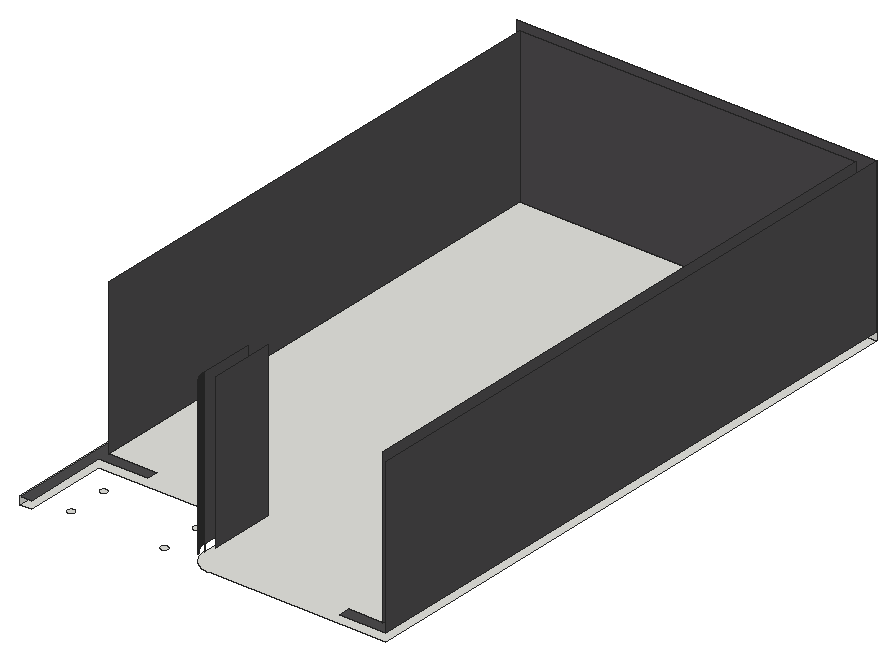
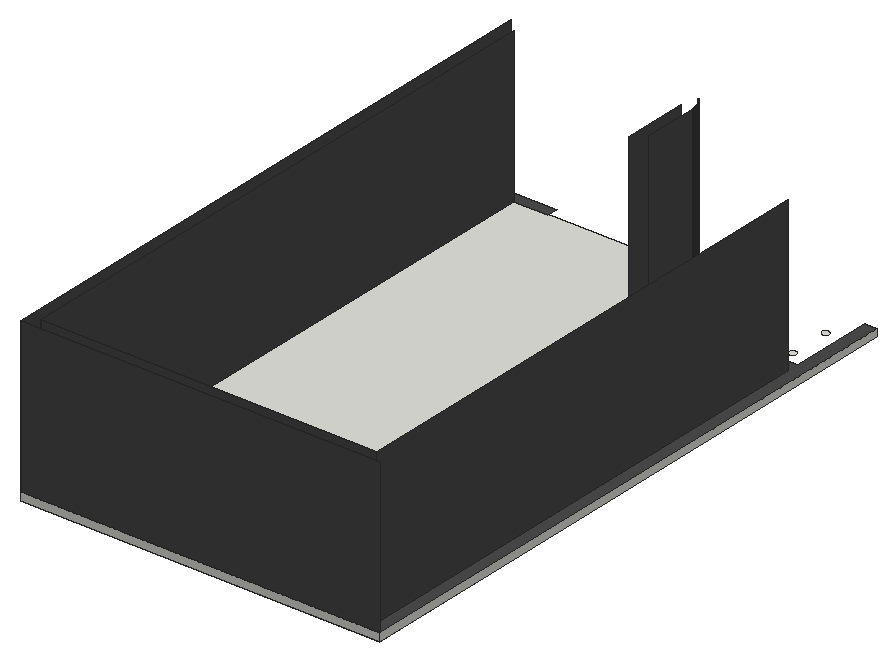
# SketchUp Ruby script. Lengths in inches.
U = 1.inch
M = Sketchup.active_model
def pt(a) = Geom::Point3d.new(a.map { |v| v * U })
def face(e, loops, mat)
  f = e.add_face(loops[0].map { |a| pt(a) })
  loops[1..].each { |l| e.add_face(l.map { |a| pt(a) }).erase! }
  f.material = f.back_material = mat if mat
  f
end
# faces: each face lists its corners as indices into pts; further lists are holes
def faces(e, pts, list, mat = nil) = list.each { |f| face(e, (f[0].is_a?(Array) ? f : [f]).map { |l| l.map { |i| pts[i] } }, mat) }
# xy, xz, yz: faces in a plane at the given z, y or x. An outline is a flat list of corners, or four numbers for a rectangle; further outlines are holes
def ring(l) = l.size == 4 ? [[l[0], l[1]], [l[2], l[1]], [l[2], l[3]], [l[0], l[3]]] : l.each_slice(2).to_a
def flat(e, list, mat, &to3) = list.each { |f| face(e, (f[0].is_a?(Array) ? f : [f]).map { |l| ring(l).map { |u, v| to3.(u, v) } }, mat) }
def xy(e, z, list, mat = nil) = flat(e, list, mat) { |x, y| [x, y, z] }
def xz(e, y, list, mat = nil) = flat(e, list, mat) { |x, z| [x, y, z] }
def yz(e, x, list, mat = nil) = flat(e, list, mat) { |y, z| [x, y, z] }
def lines(e, pts, list) = list.each { |a, b| e.add_line(pt(pts[a]), pt(pts[b])) }
# prism: a flat outline (further loops are holes) pulled along v
def prism(e, loops, v, mat = nil)
  f = face(e, loops, mat); d = Geom::Vector3d.new(v.map { |x| x * U })
  f.pushpull(f.normal.samedirection?(d) ? d.length : -d.length)
end
def box(e, o, s, mat = nil) = prism(e, [[o, [o[0] + s[0], o[1], o[2]], [o[0] + s[0], o[1] + s[1], o[2]], [o[0], o[1] + s[1], o[2]]]], [0, 0, s[2]], mat)
def at(x, y, z, deg = 0) = Geom::Transformation.translation(pt([x, y, z])) * Geom::Transformation.rotation(ORIGIN, Z_AXIS, deg.degrees)
def axes(o, x, y, z) = Geom::Transformation.new([*x, 0, *y, 0, *z, 0, *pt(o).to_a, 1])
def part(name) = M.definitions.add(name)
# library, detail: a bought-in or finely detailed component or shape, given as its bounding box
def library(name, o, s) = part(name).tap { |d| box(d.entities, o, s) }
def detail(e, o, s) = box(e.add_group.entities, o, s)
def put(e, d, t, mat = nil) = e.add_instance(d, t).tap { |i| i.material = mat if mat }
def group(e, t, mat = nil) = e.add_group.tap { |g| g.transformation = t; g.material = mat if mat }.entities
root = M.entities
M.materials.add("1423 AP 8230 BENTONITE").color = [77, 75, 77]
M.materials.add("1427 AP 686 ARMOUR-N").color = [184, 186, 189]
xy(root,119,[[37.34,197.5,37.26,197.51,37.1875,197.52,37.11,197.53,37.03,197.54,36.95,197.56,36.88,197.58,36.8,197.6,36.73,197.62,36.65,197.65,36.51,197.71,36.4375,197.74,36.37,197.77,36.09,197.93,36.03,197.98,35.97,198.02,35.91,198.07,35.79,198.18,35.73,198.23,35.68,198.29,35.57,198.41,35.52,198.47,35.48,198.53,35.43,198.59,35.27,198.87,35.24,198.9375,35.21,199.01,35.15,199.15,35.12,199.23,35.1,199.3,35.08,199.38,35.06,199.45,35.04,199.53,35.03,199.61,35.02,199.6875,35.01,199.76,35,199.84,35,200.16,35.01,200.24,35.02,200.3125,35.03,200.39,35.04,200.47,35.06,200.55,35.08,200.62,35.1,200.7,35.12,200.77,35.15,200.85,35.21,200.99,35.24,201.0625,35.27,201.13,35.43,201.41,35.48,201.47,35.52,201.53,35.57,201.59,35.68,201.71,35.73,201.77,35.79,201.82,35.91,201.93,35.97,201.98,36.03,202.02,36.09,202.07,36.37,202.23,36.4375,202.26,36.51,202.29,36.65,202.35,36.73,202.38,36.8,202.4,36.88,202.42,36.95,202.44,37.03,202.46,37.11,202.47,37.1875,202.48,37.26,202.49,37.34,202.5,37.66,202.5,37.74,202.49,37.8125,202.48,37.89,202.47,37.97,202.46,38.05,202.44,38.12,202.42,38.2,202.4,38.27,202.38,38.35,202.35,38.49,202.29,38.5625,202.26,38.63,202.23,38.91,202.07,38.97,202.02,39.03,201.98,39.09,201.93,39.21,201.82,39.27,201.77,39.32,201.71,39.43,201.59,39.48,201.53,39.52,201.47,39.57,201.41,39.73,201.13,39.76,201.0625,39.79,200.99,39.85,200.85,39.88,200.77,39.9,200.7,39.92,200.62,39.94,200.55,39.96,200.47,39.97,200.39,39.98,200.3125,39.99,200.24,40,200.16,40,199.84,39.99,199.76,39.98,199.6875,39.97,199.61,39.96,199.53,39.94,199.45,39.92,199.38,39.9,199.3,39.88,199.23,39.85,199.15,39.79,199.01,39.76,198.9375,39.73,198.87,39.57,198.59,39.52,198.53,39.48,198.47,39.43,198.41,39.32,198.29,39.27,198.23,39.21,198.18,39.09,198.07,39.03,198.02,38.97,197.98,38.91,197.93,38.63,197.77,38.5625,197.74,38.49,197.71,38.35,197.65,38.27,197.62,38.2,197.6,38.12,197.58,38.05,197.56,37.97,197.54,37.89,197.53,37.8125,197.52,37.74,197.51,37.66,197.5],[110.34,197.5,110.26,197.51,110.1875,197.52,110.11,197.53,110.03,197.54,109.95,197.56,109.88,197.58,109.8,197.6,109.73,197.62,109.65,197.65,109.51,197.71,109.4375,197.74,109.37,197.77,109.09,197.93,109.03,197.98,108.97,198.02,108.91,198.07,108.79,198.18,108.73,198.23,108.68,198.29,108.57,198.41,108.52,198.47,108.48,198.53,108.43,198.59,108.27,198.87,108.24,198.9375,108.21,199.01,108.15,199.15,108.12,199.23,108.1,199.3,108.08,199.38,108.06,199.45,108.04,199.53,108.03,199.61,108.02,199.6875,108.01,199.76,108,199.84,108,200.16,108.01,200.24,108.02,200.3125,108.03,200.39,108.04,200.47,108.06,200.55,108.08,200.62,108.1,200.7,108.12,200.77,108.15,200.85,108.21,200.99,108.24,201.0625,108.27,201.13,108.43,201.41,108.48,201.47,108.52,201.53,108.57,201.59,108.68,201.71,108.73,201.77,108.79,201.82,108.91,201.93,108.97,201.98,109.03,202.02,109.09,202.07,109.37,202.23,109.4375,202.26,109.51,202.29,109.65,202.35,109.73,202.38,109.8,202.4,109.88,202.42,109.95,202.44,110.03,202.46,110.11,202.47,110.1875,202.48,110.26,202.49,110.34,202.5,110.66,202.5,110.74,202.49,110.8125,202.48,110.89,202.47,110.97,202.46,111.05,202.44,111.12,202.42,111.2,202.4,111.27,202.38,111.35,202.35,111.49,202.29,111.5625,202.26,111.63,202.23,111.91,202.07,111.97,202.02,112.03,201.98,112.09,201.93,112.21,201.82,112.27,201.77,112.32,201.71,112.43,201.59,112.48,201.53,112.52,201.47,112.57,201.41,112.73,201.13,112.76,201.0625,112.79,200.99,112.85,200.85,112.88,200.77,112.9,200.7,112.92,200.62,112.94,200.55,112.96,200.47,112.97,200.39,112.98,200.3125,112.99,200.24,113,200.16,113,199.84,112.99,199.76,112.98,199.6875,112.97,199.61,112.96,199.53,112.94,199.45,112.92,199.38,112.9,199.3,112.88,199.23,112.85,199.15,112.79,199.01,112.76,198.9375,112.73,198.87,112.57,198.59,112.52,198.53,112.48,198.47,112.43,198.41,112.32,198.29,112.27,198.23,112.21,198.18,112.09,198.07,112.03,198.02,111.97,197.98,111.91,197.93,111.63,197.77,111.5625,197.74,111.49,197.71,111.35,197.65,111.27,197.62,111.2,197.6,111.12,197.58,111.05,197.56,110.97,197.54,110.89,197.53,110.8125,197.52,110.74,197.51,110.66,197.5],[37.34,229.5,37.26,229.51,37.1875,229.52,37.11,229.53,37.03,229.54,36.95,229.56,36.88,229.58,36.8,229.6,36.73,229.62,36.65,229.65,36.51,229.71,36.4375,229.74,36.37,229.77,36.09,229.93,36.03,229.98,35.97,230.02,35.91,230.07,35.79,230.18,35.73,230.23,35.68,230.29,35.57,230.41,35.52,230.47,35.48,230.53,35.43,230.59,35.27,230.87,35.24,230.9375,35.21,231.01,35.15,231.15,35.12,231.23,35.1,231.3,35.08,231.38,35.06,231.45,35.04,231.53,35.03,231.61,35.02,231.6875,35.01,231.76,35,231.84,35,232.16,35.01,232.24,35.02,232.3125,35.03,232.39,35.04,232.47,35.06,232.55,35.08,232.62,35.1,232.7,35.12,232.77,35.15,232.85,35.21,232.99,35.24,233.0625,35.27,233.13,35.43,233.41,35.48,233.47,35.52,233.53,35.57,233.59,35.68,233.71,35.73,233.77,35.79,233.82,35.91,233.93,35.97,233.98,36.03,234.02,36.09,234.07,36.37,234.23,36.4375,234.26,36.51,234.29,36.65,234.35,36.73,234.38,36.8,234.4,36.88,234.42,36.95,234.44,37.03,234.46,37.11,234.47,37.1875,234.48,37.26,234.49,37.34,234.5,37.66,234.5,37.74,234.49,37.8125,234.48,37.89,234.47,37.97,234.46,38.05,234.44,38.12,234.42,38.2,234.4,38.27,234.38,38.35,234.35,38.49,234.29,38.5625,234.26,38.63,234.23,38.91,234.07,38.97,234.02,39.03,233.98,39.09,233.93,39.21,233.82,39.27,233.77,39.32,233.71,39.43,233.59,39.48,233.53,39.52,233.47,39.57,233.41,39.73,233.13,39.76,233.0625,39.79,232.99,39.85,232.85,39.88,232.77,39.9,232.7,39.92,232.62,39.94,232.55,39.96,232.47,39.97,232.39,39.98,232.3125,39.99,232.24,40,232.16,40,231.84,39.99,231.76,39.98,231.6875,39.97,231.61,39.96,231.53,39.94,231.45,39.92,231.38,39.9,231.3,39.88,231.23,39.85,231.15,39.79,231.01,39.76,230.9375,39.73,230.87,39.57,230.59,39.52,230.53,39.48,230.47,39.43,230.41,39.32,230.29,39.27,230.23,39.21,230.18,39.09,230.07,39.03,230.02,38.97,229.98,38.91,229.93,38.63,229.77,38.5625,229.74,38.49,229.71,38.35,229.65,38.27,229.62,38.2,229.6,38.12,229.58,38.05,229.56,37.97,229.54,37.89,229.53,37.8125,229.52,37.74,229.51,37.66,229.5],[110.34,229.5,110.26,229.51,110.1875,229.52,110.11,229.53,110.03,229.54,109.95,229.56,109.88,229.58,109.8,229.6,109.73,229.62,109.65,229.65,109.51,229.71,109.4375,229.74,109.37,229.77,109.09,229.93,109.03,229.98,108.97,230.02,108.91,230.07,108.79,230.18,108.73,230.23,108.68,230.29,108.57,230.41,108.52,230.47,108.48,230.53,108.43,230.59,108.27,230.87,108.24,230.9375,108.21,231.01,108.15,231.15,108.12,231.23,108.1,231.3,108.08,231.38,108.06,231.45,108.04,231.53,108.03,231.61,108.02,231.6875,108.01,231.76,108,231.84,108,232.16,108.01,232.24,108.02,232.3125,108.03,232.39,108.04,232.47,108.06,232.55,108.08,232.62,108.1,232.7,108.12,232.77,108.15,232.85,108.21,232.99,108.24,233.0625,108.27,233.13,108.43,233.41,108.48,233.47,108.52,233.53,108.57,233.59,108.68,233.71,108.73,233.77,108.79,233.82,108.91,233.93,108.97,233.98,109.03,234.02,109.09,234.07,109.37,234.23,109.4375,234.26,109.51,234.29,109.65,234.35,109.73,234.38,109.8,234.4,109.88,234.42,109.95,234.44,110.03,234.46,110.11,234.47,110.1875,234.48,110.26,234.49,110.34,234.5,110.66,234.5,110.74,234.49,110.8125,234.48,110.89,234.47,110.97,234.46,111.05,234.44,111.12,234.42,111.2,234.4,111.27,234.38,111.35,234.35,111.49,234.29,111.5625,234.26,111.63,234.23,111.91,234.07,111.97,234.02,112.03,233.98,112.09,233.93,112.21,233.82,112.27,233.77,112.32,233.71,112.43,233.59,112.48,233.53,112.52,233.47,112.57,233.41,112.73,233.13,112.76,233.0625,112.79,232.99,112.85,232.85,112.88,232.77,112.9,232.7,112.92,232.62,112.94,232.55,112.96,232.47,112.97,232.39,112.98,232.3125,112.99,232.24,113,232.16,113,231.84,112.99,231.76,112.98,231.6875,112.97,231.61,112.96,231.53,112.94,231.45,112.92,231.38,112.9,231.3,112.88,231.23,112.85,231.15,112.79,231.01,112.76,230.9375,112.73,230.87,112.57,230.59,112.52,230.53,112.48,230.47,112.43,230.41,112.32,230.29,112.27,230.23,112.21,230.18,112.09,230.07,112.03,230.02,111.97,229.98,111.91,229.93,111.63,229.77,111.5625,229.74,111.49,229.71,111.35,229.65,111.27,229.62,111.2,229.6,111.12,229.58,111.05,229.56,110.97,229.54,110.89,229.53,110.8125,229.52,110.74,229.51,110.66,229.5]])
xy(root,120,[[9,186,9,672,290,672,290,192,151.78,192,151.57,192.01,151.35,192.01,150.91,192.03,150.7,192.05,150.48,192.0625,150.26,192.08,150.05,192.11,149.83,192.13,149.61,192.16,149.4,192.1875,149.18,192.22,148.97,192.26,148.76,192.29,148.54,192.34,148.12,192.42,147.9,192.47,147.69,192.52,147.48,192.58,147.27,192.63,147.0625,192.69,146.85,192.75,146.64,192.82,146.4375,192.88,146.23,192.95,146.03,193.02,145.82,193.09,145.62,193.17,145.41,193.25,145.01,193.41,144.8125,193.5,144.61,193.59,144.41,193.68,144.22,193.77,144.02,193.86,143.83,193.96,143.63,194.0625,143.44,194.16,143.25,194.27,142.875,194.48,142.6875,194.6,142.5,194.71,142.32,194.83,142.14,194.94,141.95,195.0625,141.77,195.1875,141.6,195.3125,141.42,195.4375,141.24,195.57,140.9,195.83,140.73,195.97,140.56,196.1,140.39,196.24,140.23,196.38,140.0625,196.53,139.9,196.67,139.58,196.97,139.43,197.12,139.27,197.27,139.12,197.43,138.97,197.58,138.67,197.9,138.53,198.0625,138.38,198.23,138.24,198.39,138.1,198.56,137.97,198.73,137.83,198.9,137.57,199.24,137.4375,199.42,137.3125,199.6,137.1875,199.77,137.0625,199.95,136.94,200.14,136.83,200.32,136.71,200.5,136.6,200.6875,136.48,200.875,136.27,201.25,136.16,201.44,136.0625,201.63,135.96,201.83,135.86,202.02,135.77,202.22,135.68,202.41,135.59,202.61,135.5,202.8125,135.41,203.01,135.25,203.41,135.17,203.62,135.09,203.82,135.02,204.03,134.95,204.23,134.88,204.4375,134.82,204.64,134.75,204.85,134.69,205.0625,134.63,205.27,134.58,205.48,134.52,205.69,134.47,205.9,134.42,206.12,134.34,206.54,134.29,206.76,134.26,206.97,134.22,207.18,134.1875,207.4,134.16,207.61,134.13,207.83,134.11,208.05,134.08,208.26,134.0625,208.48,134.05,208.7,134.03,208.91,134.01,209.35,134.01,209.57,134,209.78,134,252,18,252,18,186]])
xy(root,120,[[[9,186,18,186,18,252,134,252,134,209.78,134.01,209.57,134.01,209.35,134.03,208.91,134.05,208.7,134.0625,208.48,134.08,208.26,134.11,208.05,134.13,207.83,134.16,207.61,134.1875,207.4,134.22,207.18,134.26,206.97,134.29,206.76,134.34,206.54,134.42,206.12,134.47,205.9,134.52,205.69,134.58,205.48,134.63,205.27,134.69,205.0625,134.75,204.85,134.82,204.64,134.88,204.4375,134.95,204.23,135.02,204.03,135.09,203.82,135.17,203.62,135.25,203.41,135.41,203.01,135.5,202.8125,135.59,202.61,135.68,202.41,135.77,202.22,135.86,202.02,135.96,201.83,136.0625,201.63,136.16,201.44,136.27,201.25,136.48,200.875,136.6,200.6875,136.71,200.5,136.83,200.32,136.94,200.14,137.0625,199.95,137.1875,199.77,137.3125,199.6,137.4375,199.42,137.57,199.24,137.83,198.9,137.97,198.73,138.1,198.56,138.24,198.39,138.38,198.23,138.53,198.0625,138.67,197.9,138.97,197.58,139.12,197.43,139.27,197.27,139.43,197.12,139.58,196.97,139.9,196.67,140.0625,196.53,140.23,196.38,140.39,196.24,140.56,196.1,140.73,195.97,140.9,195.83,141.24,195.57,141.42,195.4375,141.6,195.3125,141.77,195.1875,141.95,195.0625,142.14,194.94,142.32,194.83,142.5,194.71,142.6875,194.6,142.875,194.48,143.25,194.27,143.44,194.16,143.63,194.0625,143.83,193.96,144.02,193.86,144.22,193.77,144.41,193.68,144.61,193.59,144.8125,193.5,145.01,193.41,145.41,193.25,145.62,193.17,145.82,193.09,146.03,193.02,146.23,192.95,146.4375,192.88,146.64,192.82,146.85,192.75,147.0625,192.69,147.27,192.63,147.48,192.58,147.69,192.52,147.9,192.47,148.12,192.42,148.54,192.34,148.76,192.29,148.97,192.26,149.18,192.22,149.4,192.1875,149.61,192.16,149.83,192.13,150.05,192.11,150.26,192.08,150.48,192.0625,150.7,192.05,150.91,192.03,151.35,192.01,151.57,192.01,151.78,192,290,192,290,672,9,672],[151.78,201,151.67,201.01,151.57,201.01,151.46,201.02,151.35,201.02,151.02,201.05,150.92,201.07,150.7,201.09,150.48,201.13,150.38,201.15,150.27,201.17,150.16,201.1875,150.06,201.21,149.95,201.24,149.85,201.26,149.74,201.29,149.64,201.32,149.53,201.35,149.43,201.375,149.32,201.41,149.12,201.47,149.01,201.51,148.91,201.55,148.81,201.58,148.71,201.625,148.61,201.66,148.51,201.71,148.31,201.79,148.21,201.84,148.11,201.88,147.91,201.98,147.82,202.03,147.72,202.08,147.625,202.13,147.53,202.1875,147.4375,202.24,147.34,202.3,147.25,202.35,146.89,202.59,146.8,202.66,146.62,202.78,146.54,202.85,146.45,202.92,146.36,202.98,146.2,203.12,146.11,203.19,146.03,203.26,145.95,203.34,145.79,203.48,145.71,203.56,145.64,203.64,145.56,203.71,145.48,203.79,145.34,203.95,145.26,204.03,145.19,204.11,145.12,204.2,144.98,204.36,144.92,204.45,144.85,204.54,144.78,204.62,144.66,204.8,144.59,204.89,144.35,205.25,144.3,205.34,144.24,205.4375,144.1875,205.53,144.13,205.625,144.08,205.72,144.03,205.82,143.98,205.91,143.88,206.11,143.84,206.21,143.79,206.31,143.71,206.51,143.66,206.61,143.625,206.71,143.58,206.81,143.55,206.91,143.51,207.01,143.47,207.12,143.41,207.32,143.375,207.43,143.35,207.53,143.32,207.64,143.29,207.74,143.26,207.85,143.24,207.95,143.21,208.06,143.1875,208.16,143.17,208.27,143.15,208.38,143.13,208.48,143.09,208.7,143.07,208.92,143.05,209.02,143.02,209.35,143.02,209.46,143.01,209.57,143.01,209.67,143,209.78,143,261,18,261,18,663,281,663,281,201]]],"1427 AP 686 ARMOUR-N")
xy(root,126,[[9,186,9,672,290,672,290,192,254,192,254,201,281,201,281,663,18,663,18,261,56,261,56,252,18,252,18,186]],"1423 AP 8230 BENTONITE")
xz(root,663,[[18,126,281,246]],"1423 AP 8230 BENTONITE")
xz(root,672,[[9,120,290,126]])
xz(root,672,[[9,126,290,246]],"1423 AP 8230 BENTONITE")
yz(root,9,[[186,120,672,126]])
yz(root,18,[[261,126,663,246]],"1423 AP 8230 BENTONITE")
yz(root,134,[[209.97,120,210,126],[209.97,120,210,126]])
yz(root,134,[[210,126,252,246]],"1423 AP 8230 BENTONITE")
yz(root,143,[[209.89,126,261,246]],"1423 AP 8230 BENTONITE")
yz(root,281,[[201,126,663,246]],"1423 AP 8230 BENTONITE")
yz(root,290,[[192,126,672,246]],"1423 AP 8230 BENTONITE")
p = [[139.27,197.27,246],[139.12,197.43,246],[139.12,197.43,126],[139.27,197.27,126],[138.97,197.58,246],[138.97,197.58,126],
  [138.82,197.74,246],[138.82,197.74,126],[138.67,197.9,246],[138.67,197.9,126],[138.53,198.0625,246],[138.53,198.0625,126],
  [138.38,198.23,246],[138.38,198.23,126],[138.24,198.39,246],[138.24,198.39,126],[138.1,198.56,246],[138.1,198.56,126],
  [137.97,198.73,246],[137.97,198.73,126],[137.83,198.9,246],[137.83,198.9,126],[137.7,199.07,246],[137.7,199.07,126],
  [137.57,199.24,246],[137.57,199.24,126],[137.4375,199.42,246],[137.4375,199.42,126],[137.3125,199.6,246],[137.3125,199.6,126],
  [137.1875,199.77,246],[137.1875,199.77,126],[137.0625,199.95,246],[137.0625,199.95,126],[136.94,200.14,246],[136.94,200.14,126],
  [136.83,200.32,246],[136.83,200.32,126],[136.71,200.5,246],[136.71,200.5,126],[136.6,200.6875,246],[136.6,200.6875,126],
  [136.48,200.875,246],[136.48,200.875,126],[136.375,201.0625,246],[136.375,201.0625,126],[136.27,201.25,246],[136.27,201.25,126],
  [136.16,201.44,246],[136.16,201.44,126],[136.0625,201.63,246],[136.0625,201.63,126],[135.96,201.83,246],[135.96,201.83,126],
  [135.86,202.02,246],[135.86,202.02,126],[135.77,202.22,246],[135.77,202.22,126],[135.68,202.41,246],[135.68,202.41,126],
  [135.59,202.61,246],[135.59,202.61,126],[135.5,202.8125,246],[135.5,202.8125,126],[135.41,203.01,246],[135.41,203.01,126],
  [135.33,203.21,246],[135.33,203.21,126],[135.25,203.41,246],[135.25,203.41,126],[135.17,203.62,246],[135.17,203.62,126],
  [135.09,203.82,246],[135.09,203.82,126],[135.02,204.03,246],[135.02,204.03,126],[134.95,204.23,246],[134.95,204.23,126],
  [134.88,204.4375,246],[134.88,204.4375,126],[134.82,204.64,246],[134.82,204.64,126],[134.75,204.85,246],[134.75,204.85,126],
  [134.69,205.0625,246],[134.69,205.0625,126],[134.63,205.27,246],[134.63,205.27,126],[134.58,205.48,246],[134.58,205.48,126],
  [134.52,205.69,246],[134.52,205.69,126],[134.47,205.9,246],[134.47,205.9,126],[134.42,206.12,246],[134.42,206.12,126],
  [134.38,206.33,246],[134.38,206.33,126],[134.34,206.54,246],[134.34,206.54,126],[134.29,206.76,246],[134.29,206.76,126],
  [134.26,206.97,246],[134.26,206.97,126],[134.22,207.18,246],[134.22,207.18,126],[134.1875,207.4,246],[134.1875,207.4,126],
  [134.16,207.61,246],[134.16,207.61,126],[134.13,207.83,246],[134.13,207.83,126],[134.11,208.05,246],[134.11,208.05,126],
  [134.08,208.26,246],[134.08,208.26,126],[134.0625,208.48,246],[134.0625,208.48,126],[134.05,208.7,246],[134.05,208.7,126]]
faces(root,p,[[0,1,2,3],[1,4,5,2],[4,6,7,5],[6,8,9,7],[8,10,11,9],[10,12,13,11],[12,14,15,13],[14,16,17,15],
  [16,18,19,17],[18,20,21,19],[20,22,23,21],[22,24,25,23],[24,26,27,25],[26,28,29,27],[28,30,31,29],[30,32,33,31],
  [32,34,35,33],[34,36,37,35],[36,38,39,37],[38,40,41,39],[40,42,43,41],[42,44,45,43],[44,46,47,45],[46,48,49,47],
  [48,50,51,49],[50,52,53,51],[52,54,55,53],[54,56,57,55],[56,58,59,57],[58,60,61,59],[60,62,63,61],[62,64,65,63],
  [64,66,67,65],[66,68,69,67],[68,70,71,69],[70,72,73,71],[72,74,75,73],[74,76,77,75],[76,78,79,77],[78,80,81,79],
  [80,82,83,81],[82,84,85,83],[84,86,87,85],[86,88,89,87],[88,90,91,89],[90,92,93,91],[92,94,95,93],[94,96,97,95],
  [96,98,99,97],[98,100,101,99],[100,102,103,101],[102,104,105,103],[104,106,107,105],[106,108,109,107],[108,110,111,109],[110,112,113,111],
  [112,114,115,113],[114,116,117,115],[116,118,119,117]],"1423 AP 8230 BENTONITE")
